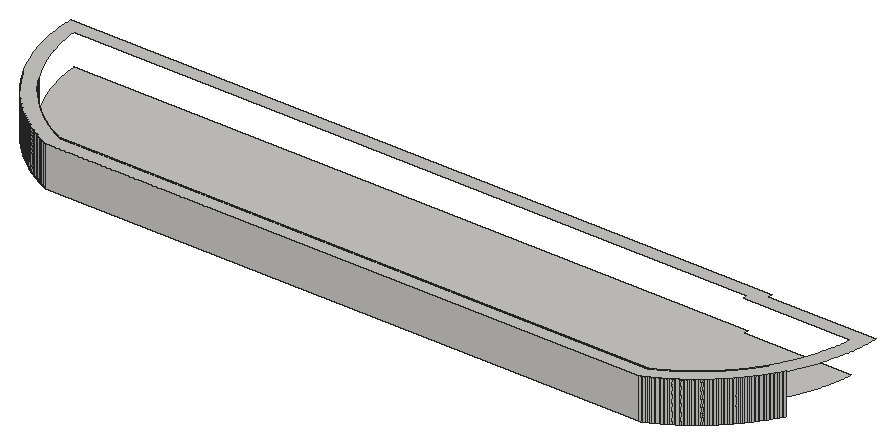
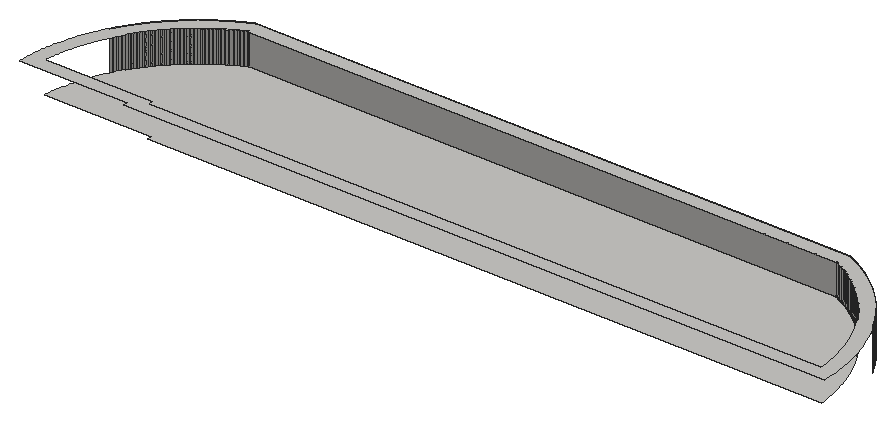
# SketchUp Ruby script. Lengths in inches.
U = 1.inch
M = Sketchup.active_model
def pt(a) = Geom::Point3d.new(a.map { |v| v * U })
def face(e, loops, mat)
  f = e.add_face(loops[0].map { |a| pt(a) })
  loops[1..].each { |l| e.add_face(l.map { |a| pt(a) }).erase! }
  f.material = f.back_material = mat if mat
  f
end
# faces: each face lists its corners as indices into pts; further lists are holes
def faces(e, pts, list, mat = nil) = list.each { |f| face(e, (f[0].is_a?(Array) ? f : [f]).map { |l| l.map { |i| pts[i] } }, mat) }
# xy, xz, yz: faces in a plane at the given z, y or x. An outline is a flat list of corners, or four numbers for a rectangle; further outlines are holes
def ring(l) = l.size == 4 ? [[l[0], l[1]], [l[2], l[1]], [l[2], l[3]], [l[0], l[3]]] : l.each_slice(2).to_a
def flat(e, list, mat, &to3) = list.each { |f| face(e, (f[0].is_a?(Array) ? f : [f]).map { |l| ring(l).map { |u, v| to3.(u, v) } }, mat) }
def xy(e, z, list, mat = nil) = flat(e, list, mat) { |x, y| [x, y, z] }
def xz(e, y, list, mat = nil) = flat(e, list, mat) { |x, z| [x, y, z] }
def yz(e, x, list, mat = nil) = flat(e, list, mat) { |y, z| [x, y, z] }
def lines(e, pts, list) = list.each { |a, b| e.add_line(pt(pts[a]), pt(pts[b])) }
# prism: a flat outline (further loops are holes) pulled along v
def prism(e, loops, v, mat = nil)
  f = face(e, loops, mat); d = Geom::Vector3d.new(v.map { |x| x * U })
  f.pushpull(f.normal.samedirection?(d) ? d.length : -d.length)
end
def box(e, o, s, mat = nil) = prism(e, [[o, [o[0] + s[0], o[1], o[2]], [o[0] + s[0], o[1] + s[1], o[2]], [o[0], o[1] + s[1], o[2]]]], [0, 0, s[2]], mat)
def at(x, y, z, deg = 0) = Geom::Transformation.translation(pt([x, y, z])) * Geom::Transformation.rotation(ORIGIN, Z_AXIS, deg.degrees)
def axes(o, x, y, z) = Geom::Transformation.new([*x, 0, *y, 0, *z, 0, *pt(o).to_a, 1])
def part(name) = M.definitions.add(name)
# library, detail: a bought-in or finely detailed component or shape, given as its bounding box
def library(name, o, s) = part(name).tap { |d| box(d.entities, o, s) }
def detail(e, o, s) = box(e.add_group.entities, o, s)
def put(e, d, t, mat = nil) = e.add_instance(d, t).tap { |i| i.material = mat if mat }
def group(e, t, mat = nil) = e.add_group.tap { |g| g.transformation = t; g.material = mat if mat }.entities
root = M.entities
M.materials.add("[Stone Sandstone Ashlar Light]").color = [201, 199, 196]
xy(root,-10,[[240.65,3,371.35,3,371.43,3.04,371.76,3.19,372.4,3.51,372.72,3.68,373.04,3.84,373.36,4.01,373.67,4.1875,373.99,4.36,374.61,4.72,375.23,5.1,375.83,5.48,376.14,5.68,376.43,5.875,376.73,6.08,377.03,6.28,377.61,6.7,377.9,6.92,378.19,7.13,378.48,7.35,378.76,7.57,379.6,8.26,380.14,8.72,380.95,9.44,381.21,9.69,381.47,9.9375,381.73,10.1875,381.98,10.44,382.24,10.7,382.74,11.22,382.98,11.48,383.23,11.74,383.71,12.28,383.94,12.55,384.17,12.83,384.4,13.1,384.86,13.66,385.08,13.94,385.52,14.52,385.73,14.8,385.94,15.1,386.36,15.68,386.96,16.58,387.15,16.88,387.34,17.1875,387.53,17.5,387.72,17.8,387.9,18.11,388.08,18.43,388.26,18.74,388.43,19.05,388.77,19.69,389.25,20.65,389.41,20.98,389.56,21.31,389.71,21.63,389.85,21.96,390,22.29,390.14,22.625,390.27,22.96,390.41,23.29,390.54,23.625,390.66,23.96,390.79,24.3,390.91,24.64,391.02,24.98,391.14,25.32,391.25,25.67,391.35,26.01,391.46,26.35,391.66,27.05,391.75,27.39,391.93,28.09,392.17,29.14,392.24,29.49,392.3125,29.85,392.38,30.2,392.44,30.56,392.5,30.91,392.56,31.27,392.61,31.62,392.66,31.98,392.71,32.33,392.75,32.69,392.79,33,369,33,369,34,219.12,34,219.14,33.77,219.17,33.41,219.29,32.33,219.34,31.98,219.39,31.62,219.44,31.27,219.5,30.91,219.56,30.56,219.62,30.2,219.6875,29.85,219.76,29.49,219.83,29.14,220.07,28.09,220.25,27.39,220.34,27.05,220.54,26.35,220.65,26.01,220.75,25.67,220.86,25.32,220.98,24.98,221.09,24.64,221.21,24.3,221.34,23.96,221.46,23.625,221.59,23.29,221.73,22.96,221.86,22.625,222,22.29,222.15,21.96,222.29,21.63,222.44,21.31,222.59,20.98,222.75,20.65,223.23,19.69,223.57,19.05,223.74,18.74,223.92,18.43,224.1,18.11,224.28,17.8,224.47,17.5,224.66,17.1875,224.85,16.88,225.04,16.58,225.64,15.68,226.06,15.1,226.27,14.8,226.48,14.52,226.92,13.94,227.14,13.66,227.6,13.1,227.83,12.83,228.06,12.55,228.29,12.28,228.77,11.74,229.02,11.48,229.26,11.22,229.76,10.7,230.02,10.44,230.27,10.1875,230.53,9.9375,230.79,9.69,231.05,9.44,231.86,8.72,232.4,8.26,233.24,7.57,233.52,7.35,233.81,7.13,234.1,6.92,234.39,6.7,234.97,6.28,235.27,6.08,235.57,5.875,235.86,5.68,236.17,5.48,236.77,5.1,237.39,4.72,238.01,4.36,238.33,4.1875,238.64,4.01,238.96,3.84,239.28,3.68,239.6,3.51,240.24,3.19,240.57,3.04]],"[Stone Sandstone Ashlar Light]")
xy(root,-3,[[[240,0,372,0,372.35,0.16,372.71,0.32,373.41,0.66,373.75,0.83,374.1,1.01,374.44,1.19,374.79,1.375,375.47,1.75,375.8,1.95,376.14,2.14,376.8,2.54,377.79,3.17,379.07,4.05,379.38,4.28,379.7,4.51,380.01,4.74,380.3125,4.98,380.62,5.22,380.92,5.46,381.82,6.21,382.11,6.46,382.41,6.72,382.69,6.98,382.98,7.24,383.27,7.51,383.55,7.77,384.1,8.32,384.375,8.59,384.65,8.87,384.92,9.15,385.18,9.4375,385.44,9.72,385.96,10.3,386.22,10.6,386.47,10.89,386.72,11.19,386.96,11.49,387.21,11.79,387.45,12.1,387.68,12.41,387.92,12.72,388.38,13.34,388.6,13.66,388.83,13.98,389.05,14.3,389.47,14.95,389.68,15.28,389.89,15.6,390.09,15.9375,390.3,16.27,390.49,16.6,390.6875,16.94,390.88,17.28,391.06,17.62,391.25,17.96,391.43,18.31,391.61,18.65,392.12,19.7,392.28,20.05,392.45,20.4,392.6,20.76,392.76,21.12,392.91,21.47,393.05,21.83,393.2,22.2,393.48,22.92,393.61,23.29,393.74,23.65,393.86,24.02,393.99,24.39,394.11,24.76,394.33,25.5,394.55,26.25,394.75,27,394.93,27.76,395.02,28.13,395.18,28.89,395.26,29.28,395.4,30.04,395.46,30.42,395.52,30.81,395.58,31.19,395.64,31.58,395.69,31.96,395.73,32.35,395.77,32.73,395.8125,33.12,395.85,33.51,395.88,33.89,395.91,34.28,395.97,35.45,395.98,35.83,395.99,36,372,36,372,37,216,37,216,36.61,216.02,35.83,216.03,35.45,216.09,34.28,216.12,33.89,216.15,33.51,216.1875,33.12,216.23,32.73,216.27,32.35,216.31,31.96,216.36,31.58,216.42,31.19,216.48,30.81,216.54,30.42,216.6,30.04,216.74,29.28,216.82,28.89,216.98,28.13,217.07,27.76,217.25,27,217.45,26.25,217.67,25.5,217.89,24.76,218.01,24.39,218.14,24.02,218.26,23.65,218.39,23.29,218.52,22.92,218.8,22.2,218.95,21.83,219.09,21.47,219.24,21.12,219.4,20.76,219.55,20.4,219.72,20.05,219.88,19.7,220.39,18.65,220.57,18.31,220.75,17.96,220.94,17.62,221.12,17.28,221.3125,16.94,221.51,16.6,221.7,16.27,221.91,15.9375,222.11,15.6,222.32,15.28,222.53,14.95,222.95,14.3,223.17,13.98,223.4,13.66,223.62,13.34,224.08,12.72,224.32,12.41,224.55,12.1,224.79,11.79,225.04,11.49,225.28,11.19,225.53,10.89,225.78,10.6,226.04,10.3,226.56,9.72,226.82,9.4375,227.08,9.15,227.35,8.87,227.625,8.59,227.9,8.32,228.45,7.77,228.73,7.51,229.02,7.24,229.31,6.98,229.59,6.72,229.89,6.46,230.18,6.21,231.08,5.46,231.38,5.22,231.6875,4.98,231.99,4.74,232.3,4.51,232.62,4.28,232.93,4.05,234.21,3.17,235.2,2.54,235.86,2.14,236.2,1.95,236.53,1.75,237.21,1.375,237.56,1.19,237.9,1.01,238.25,0.83,238.59,0.66,239.29,0.32,239.65,0.16],[240.65,3,240.57,3.04,240.24,3.19,239.6,3.51,239.28,3.68,238.96,3.84,238.64,4.01,238.33,4.1875,238.01,4.36,237.39,4.72,236.77,5.1,236.17,5.48,235.86,5.68,235.57,5.875,235.27,6.08,234.97,6.28,234.39,6.7,234.1,6.92,233.81,7.13,233.52,7.35,233.24,7.57,232.4,8.26,231.86,8.72,231.05,9.44,230.79,9.69,230.53,9.9375,230.27,10.1875,230.02,10.44,229.76,10.7,229.26,11.22,229.02,11.48,228.77,11.74,228.29,12.28,228.06,12.55,227.83,12.83,227.6,13.1,227.14,13.66,226.92,13.94,226.48,14.52,226.27,14.8,226.06,15.1,225.64,15.68,225.04,16.58,224.85,16.88,224.66,17.1875,224.47,17.5,224.28,17.8,224.1,18.11,223.92,18.43,223.74,18.74,223.57,19.05,223.23,19.69,222.75,20.65,222.59,20.98,222.44,21.31,222.29,21.63,222.15,21.96,222,22.29,221.86,22.625,221.73,22.96,221.59,23.29,221.46,23.625,221.34,23.96,221.21,24.3,221.09,24.64,220.98,24.98,220.86,25.32,220.75,25.67,220.65,26.01,220.54,26.35,220.34,27.05,220.25,27.39,220.07,28.09,219.83,29.14,219.76,29.49,219.6875,29.85,219.62,30.2,219.56,30.56,219.5,30.91,219.44,31.27,219.39,31.62,219.34,31.98,219.29,32.33,219.17,33.41,219.14,33.77,219.12,34,369,34,369,33,392.79,33,392.75,32.69,392.71,32.33,392.66,31.98,392.61,31.62,392.56,31.27,392.5,30.91,392.44,30.56,392.38,30.2,392.3125,29.85,392.24,29.49,392.17,29.14,391.93,28.09,391.75,27.39,391.66,27.05,391.46,26.35,391.35,26.01,391.25,25.67,391.14,25.32,391.02,24.98,390.91,24.64,390.79,24.3,390.66,23.96,390.54,23.625,390.41,23.29,390.27,22.96,390.14,22.625,390,22.29,389.85,21.96,389.71,21.63,389.56,21.31,389.41,20.98,389.25,20.65,388.77,19.69,388.43,19.05,388.26,18.74,388.08,18.43,387.9,18.11,387.72,17.8,387.53,17.5,387.34,17.1875,387.15,16.88,386.96,16.58,386.36,15.68,385.94,15.1,385.73,14.8,385.52,14.52,385.08,13.94,384.86,13.66,384.4,13.1,384.17,12.83,383.94,12.55,383.71,12.28,383.23,11.74,382.98,11.48,382.74,11.22,382.24,10.7,381.98,10.44,381.73,10.1875,381.47,9.9375,381.21,9.69,380.95,9.44,380.14,8.72,379.6,8.26,378.76,7.57,378.48,7.35,378.19,7.13,377.9,6.92,377.61,6.7,377.03,6.28,376.73,6.08,376.43,5.875,376.14,5.68,375.83,5.48,375.23,5.1,374.61,4.72,373.99,4.36,373.67,4.1875,373.36,4.01,373.04,3.84,372.72,3.68,372.4,3.51,371.76,3.19,371.43,3.04,371.35,3]]],"[Stone Sandstone Ashlar Light]")
xz(root,0,[[240,-12,372,-3]],"[Stone Sandstone Ashlar Light]")
xz(root,3,[[240.65,-10,371.35,-3]],"[Stone Sandstone Ashlar Light]")
p = [[240,0,-3],[239.65,0.16,-3],[239.65,0.16,-12],[240,0,-12],[372.35,0.16,-3],[372,0,-3],
  [372,0,-12],[372.35,0.16,-12],[239.29,0.32,-3],[239.29,0.32,-12],[372.71,0.32,-3],[372.71,0.32,-12],
  [238.94,0.49,-3],[238.94,0.49,-12],[373.06,0.49,-3],[373.06,0.49,-12],[238.59,0.66,-3],[238.59,0.66,-12],
  [373.41,0.66,-3],[373.41,0.66,-12],[238.25,0.83,-3],[238.25,0.83,-12],[373.75,0.83,-3],[373.75,0.83,-12],
  [237.9,1.01,-3],[237.9,1.01,-12],[374.1,1.01,-3],[374.1,1.01,-12],[237.56,1.19,-3],[237.56,1.19,-12],
  [374.44,1.19,-3],[374.44,1.19,-12],[237.21,1.375,-3],[237.21,1.375,-12],[374.79,1.375,-3],[374.79,1.375,-12],
  [236.87,1.5625,-3],[236.87,1.5625,-12],[375.13,1.5625,-3],[375.13,1.5625,-12],[236.53,1.75,-3],[236.53,1.75,-12],
  [375.47,1.75,-3],[375.47,1.75,-12],[236.2,1.95,-3],[236.2,1.95,-12],[375.8,1.95,-3],[375.8,1.95,-12],
  [235.86,2.14,-3],[235.86,2.14,-12],[376.14,2.14,-3],[376.14,2.14,-12],[235.53,2.34,-3],[235.53,2.34,-12],
  [376.47,2.34,-3],[376.47,2.34,-12],[235.2,2.54,-3],[235.2,2.54,-12],[376.8,2.54,-3],[376.8,2.54,-12],
  [234.87,2.75,-3],[234.87,2.75,-12],[377.13,2.75,-3],[377.13,2.75,-12],[234.54,2.96,-3],[234.54,2.96,-12],
  [377.46,2.96,-3],[377.46,2.96,-12],[234.21,3.17,-3],[234.21,3.17,-12],[377.79,3.17,-3],[377.79,3.17,-12],
  [233.89,3.39,-3],[233.89,3.39,-12],[378.11,3.39,-3],[378.11,3.39,-12],[233.57,3.61,-3],[233.57,3.61,-12],
  [378.43,3.61,-3],[378.43,3.61,-12],[233.25,3.83,-3],[233.25,3.83,-12],[378.75,3.83,-3],[378.75,3.83,-12],
  [232.93,4.05,-3],[232.93,4.05,-12],[379.07,4.05,-3],[379.07,4.05,-12],[232.62,4.28,-3],[232.62,4.28,-12],
  [379.38,4.28,-3],[379.38,4.28,-12],[232.3,4.51,-3],[232.3,4.51,-12],[379.7,4.51,-3],[379.7,4.51,-12],
  [231.99,4.74,-3],[231.99,4.74,-12],[380.01,4.74,-3],[380.01,4.74,-12],[231.6875,4.98,-3],[231.6875,4.98,-12],
  [380.3125,4.98,-3],[380.3125,4.98,-12],[231.38,5.22,-3],[231.38,5.22,-12],[380.62,5.22,-3],[380.62,5.22,-12],
  [231.08,5.46,-3],[231.08,5.46,-12],[380.92,5.46,-3],[380.92,5.46,-12],[230.78,5.71,-3],[230.78,5.71,-12],
  [381.22,5.71,-3],[381.22,5.71,-12],[230.48,5.96,-3],[230.48,5.96,-12],[381.52,5.96,-3],[381.52,5.96,-12],
  [230.18,6.21,-3],[230.18,6.21,-12],[381.82,6.21,-3],[381.82,6.21,-12],[229.89,6.46,-3],[229.89,6.46,-12],
  [382.11,6.46,-3],[382.11,6.46,-12],[229.59,6.72,-3],[229.59,6.72,-12],[382.41,6.72,-3],[382.41,6.72,-12],
  [229.31,6.98,-3],[229.31,6.98,-12],[382.69,6.98,-3],[382.69,6.98,-12],[229.02,7.24,-3],[229.02,7.24,-12],
  [382.98,7.24,-3],[382.98,7.24,-12],[228.73,7.51,-3],[228.73,7.51,-12],[383.27,7.51,-3],[383.27,7.51,-12],
  [228.45,7.77,-3],[228.45,7.77,-12],[383.55,7.77,-3],[383.55,7.77,-12],[228.17,8.05,-3],[228.17,8.05,-12],
  [383.83,8.05,-3],[383.83,8.05,-12],[227.9,8.32,-3],[227.9,8.32,-12],[384.1,8.32,-3],[384.1,8.32,-12],
  [227.625,8.59,-3],[227.625,8.59,-12],[384.375,8.59,-3],[384.375,8.59,-12],[227.35,8.87,-3],[227.35,8.87,-12],
  [384.65,8.87,-3],[384.65,8.87,-12],[227.08,9.15,-3],[227.08,9.15,-12],[384.92,9.15,-3],[384.92,9.15,-12],
  [226.82,9.4375,-3],[226.82,9.4375,-12],[385.18,9.4375,-3],[385.18,9.4375,-12],[226.56,9.72,-3],[226.56,9.72,-12],
  [385.44,9.72,-3],[385.44,9.72,-12],[226.3,10.01,-3],[226.3,10.01,-12],[385.7,10.01,-3],[385.7,10.01,-12],
  [226.04,10.3,-3],[226.04,10.3,-12],[385.96,10.3,-3],[385.96,10.3,-12],[225.78,10.6,-3],[225.78,10.6,-12],
  [386.22,10.6,-3],[386.22,10.6,-12],[225.53,10.89,-3],[225.53,10.89,-12],[386.47,10.89,-3],[386.47,10.89,-12],
  [225.28,11.19,-3],[225.28,11.19,-12],[386.72,11.19,-3],[386.72,11.19,-12],[225.04,11.49,-3],[225.04,11.49,-12],
  [386.96,11.49,-3],[386.96,11.49,-12],[224.79,11.79,-3],[224.79,11.79,-12],[387.21,11.79,-3],[387.21,11.79,-12],
  [224.55,12.1,-3],[224.55,12.1,-12],[387.45,12.1,-3],[387.45,12.1,-12],[224.32,12.41,-3],[224.32,12.41,-12],
  [387.68,12.41,-3],[387.68,12.41,-12],[224.08,12.72,-3],[224.08,12.72,-12],[387.92,12.72,-3],[387.92,12.72,-12],
  [223.85,13.03,-3],[223.85,13.03,-12],[388.15,13.03,-3],[388.15,13.03,-12],[223.62,13.34,-3],[223.62,13.34,-12],
  [388.38,13.34,-3],[388.38,13.34,-12],[223.4,13.66,-3],[223.4,13.66,-12],[388.6,13.66,-3],[388.6,13.66,-12],
  [223.17,13.98,-3],[223.17,13.98,-12],[388.83,13.98,-3],[388.83,13.98,-12],[222.95,14.3,-3],[222.95,14.3,-12],
  [389.05,14.3,-3],[389.05,14.3,-12],[222.74,14.625,-3],[222.74,14.625,-12],[389.26,14.625,-3],[389.26,14.625,-12],
  [222.53,14.95,-3],[222.53,14.95,-12],[389.47,14.95,-3],[389.47,14.95,-12],[222.32,15.28,-3],[222.32,15.28,-12],
  [389.68,15.28,-3],[389.68,15.28,-12],[222.11,15.6,-3],[222.11,15.6,-12],[389.89,15.6,-3],[389.89,15.6,-12],
  [221.91,15.9375,-3],[221.91,15.9375,-12],[390.09,15.9375,-3],[390.09,15.9375,-12],[221.7,16.27,-3],[221.7,16.27,-12],
  [390.3,16.27,-3],[390.3,16.27,-12],[221.51,16.6,-3],[221.51,16.6,-12],[390.49,16.6,-3],[390.49,16.6,-12],
  [221.3125,16.94,-3],[221.3125,16.94,-12],[390.6875,16.94,-3],[390.6875,16.94,-12],[221.12,17.28,-3],[221.12,17.28,-12],
  [390.88,17.28,-3],[390.88,17.28,-12],[240.24,3.19,-3],[240.57,3.04,-3],[240.57,3.04,-10],[240.24,3.19,-10],
  [240.65,3,-3],[240.65,3,-10],[371.35,3,-3],[371.43,3.04,-3],[371.43,3.04,-10],[371.35,3,-10],
  [371.76,3.19,-3],[371.76,3.19,-10],[239.92,3.35,-3],[239.92,3.35,-10],[372.08,3.35,-3],[372.08,3.35,-10],
  [239.6,3.51,-3],[239.6,3.51,-10],[372.4,3.51,-3],[372.4,3.51,-10],[239.28,3.68,-3],[239.28,3.68,-10],
  [372.72,3.68,-3],[372.72,3.68,-10],[238.96,3.84,-3],[238.96,3.84,-10],[373.04,3.84,-3],[373.04,3.84,-10],
  [238.64,4.01,-3],[238.64,4.01,-10],[373.36,4.01,-3],[373.36,4.01,-10],[238.33,4.1875,-3],[238.33,4.1875,-10],
  [373.67,4.1875,-3],[373.67,4.1875,-10],[238.01,4.36,-3],[238.01,4.36,-10],[373.99,4.36,-3],[373.99,4.36,-10],
  [237.7,4.54,-3],[237.7,4.54,-10],[374.3,4.54,-3],[374.3,4.54,-10],[237.39,4.72,-3],[237.39,4.72,-10],
  [374.61,4.72,-3],[374.61,4.72,-10],[237.08,4.91,-3],[237.08,4.91,-10],[374.92,4.91,-3],[374.92,4.91,-10],
  [236.77,5.1,-3],[236.77,5.1,-10],[375.23,5.1,-3],[375.23,5.1,-10],[236.47,5.29,-3],[236.47,5.29,-10],
  [375.53,5.29,-3],[375.53,5.29,-10],[236.17,5.48,-3],[236.17,5.48,-10],[375.83,5.48,-3],[375.83,5.48,-10],
  [235.86,5.68,-3],[235.86,5.68,-10],[376.14,5.68,-3],[376.14,5.68,-10],[235.57,5.875,-3],[235.57,5.875,-10],
  [376.43,5.875,-3],[376.43,5.875,-10],[235.27,6.08,-3],[235.27,6.08,-10],[376.73,6.08,-3],[376.73,6.08,-10],
  [234.97,6.28,-3],[234.97,6.28,-10],[377.03,6.28,-3],[377.03,6.28,-10],[234.68,6.49,-3],[234.68,6.49,-10],
  [377.32,6.49,-3],[377.32,6.49,-10],[234.39,6.7,-3],[234.39,6.7,-10],[377.61,6.7,-3],[377.61,6.7,-10],
  [234.1,6.92,-3],[234.1,6.92,-10],[377.9,6.92,-3],[377.9,6.92,-10],[233.81,7.13,-3],[233.81,7.13,-10],
  [378.19,7.13,-3],[378.19,7.13,-10],[233.52,7.35,-3],[233.52,7.35,-10],[378.48,7.35,-3],[378.48,7.35,-10],
  [233.24,7.57,-3],[233.24,7.57,-10],[378.76,7.57,-3],[378.76,7.57,-10],[232.96,7.8,-3],[232.96,7.8,-10],
  [379.04,7.8,-3],[379.04,7.8,-10],[232.68,8.03,-3],[232.68,8.03,-10],[379.32,8.03,-3],[379.32,8.03,-10],
  [232.4,8.26,-3],[232.4,8.26,-10],[379.6,8.26,-3],[379.6,8.26,-10],[232.13,8.49,-3],[232.13,8.49,-10],
  [379.87,8.49,-3],[379.87,8.49,-10],[231.86,8.72,-3],[231.86,8.72,-10],[380.14,8.72,-3],[380.14,8.72,-10],
  [231.59,8.96,-3],[231.59,8.96,-10],[380.41,8.96,-3],[380.41,8.96,-10],[231.32,9.2,-3],[231.32,9.2,-10],
  [380.68,9.2,-3],[380.68,9.2,-10],[231.05,9.44,-3],[231.05,9.44,-10],[380.95,9.44,-3],[380.95,9.44,-10],
  [230.79,9.69,-3],[230.79,9.69,-10],[381.21,9.69,-3],[381.21,9.69,-10],[230.53,9.9375,-3],[230.53,9.9375,-10],
  [381.47,9.9375,-3],[381.47,9.9375,-10],[230.27,10.1875,-3],[230.27,10.1875,-10],[381.73,10.1875,-3],[381.73,10.1875,-10],
  [230.02,10.44,-3],[230.02,10.44,-10],[381.98,10.44,-3],[381.98,10.44,-10],[229.76,10.7,-3],[229.76,10.7,-10],
  [382.24,10.7,-3],[382.24,10.7,-10],[229.51,10.96,-3],[229.51,10.96,-10],[382.49,10.96,-3],[382.49,10.96,-10],
  [229.26,11.22,-3],[229.26,11.22,-10],[382.74,11.22,-3],[382.74,11.22,-10],[229.02,11.48,-3],[229.02,11.48,-10],
  [382.98,11.48,-3],[382.98,11.48,-10],[228.77,11.74,-3],[228.77,11.74,-10],[383.23,11.74,-3],[383.23,11.74,-10],
  [228.53,12.01,-3],[228.53,12.01,-10],[383.47,12.01,-3],[383.47,12.01,-10],[228.29,12.28,-3],[228.29,12.28,-10],
  [383.71,12.28,-3],[383.71,12.28,-10],[228.06,12.55,-3],[228.06,12.55,-10],[383.94,12.55,-3],[383.94,12.55,-10],
  [227.83,12.83,-3],[227.83,12.83,-10],[384.17,12.83,-3],[384.17,12.83,-10],[227.6,13.1,-3],[227.6,13.1,-10],
  [384.4,13.1,-3],[384.4,13.1,-10],[227.37,13.38,-3],[227.37,13.38,-10],[384.63,13.38,-3],[384.63,13.38,-10],
  [227.14,13.66,-3],[227.14,13.66,-10],[384.86,13.66,-3],[384.86,13.66,-10],[226.92,13.94,-3],[226.92,13.94,-10],
  [385.08,13.94,-3],[385.08,13.94,-10],[226.7,14.23,-3],[226.7,14.23,-10],[385.3,14.23,-3],[385.3,14.23,-10],
  [226.48,14.52,-3],[226.48,14.52,-10],[385.52,14.52,-3],[385.52,14.52,-10],[226.27,14.8,-3],[226.27,14.8,-10],
  [385.73,14.8,-3],[385.73,14.8,-10],[226.06,15.1,-3],[226.06,15.1,-10],[385.94,15.1,-3],[385.94,15.1,-10],
  [225.85,15.39,-3],[225.85,15.39,-10],[386.15,15.39,-3],[386.15,15.39,-10],[225.64,15.68,-3],[225.64,15.68,-10],
  [386.36,15.68,-3],[386.36,15.68,-10],[225.44,15.98,-3],[225.44,15.98,-10],[386.56,15.98,-3],[386.56,15.98,-10],
  [225.24,16.28,-3],[225.24,16.28,-10],[386.76,16.28,-3],[386.76,16.28,-10],[225.04,16.58,-3],[225.04,16.58,-10],
  [386.96,16.58,-3],[386.96,16.58,-10],[224.85,16.88,-3],[224.85,16.88,-10],[387.15,16.88,-3],[387.15,16.88,-10],
  [224.66,17.1875,-3],[224.66,17.1875,-10],[387.34,17.1875,-3],[387.34,17.1875,-10]]
faces(root,p,[[0,1,2,3],[4,5,6,7],[1,8,9,2],[10,4,7,11],[8,12,13,9],[14,10,11,15],[12,16,17,13],[18,14,15,19],
  [16,20,21,17],[22,18,19,23],[20,24,25,21],[26,22,23,27],[24,28,29,25],[30,26,27,31],[28,32,33,29],[34,30,31,35],
  [32,36,37,33],[38,34,35,39],[36,40,41,37],[42,38,39,43],[40,44,45,41],[46,42,43,47],[44,48,49,45],[50,46,47,51],
  [48,52,53,49],[54,50,51,55],[52,56,57,53],[58,54,55,59],[56,60,61,57],[62,58,59,63],[60,64,65,61],[66,62,63,67],
  [64,68,69,65],[70,66,67,71],[68,72,73,69],[74,70,71,75],[72,76,77,73],[78,74,75,79],[76,80,81,77],[82,78,79,83],
  [80,84,85,81],[86,82,83,87],[84,88,89,85],[90,86,87,91],[88,92,93,89],[94,90,91,95],[92,96,97,93],[98,94,95,99],
  [96,100,101,97],[102,98,99,103],[100,104,105,101],[106,102,103,107],[104,108,109,105],[110,106,107,111],[108,112,113,109],[114,110,111,115],
  [112,116,117,113],[118,114,115,119],[116,120,121,117],[122,118,119,123],[120,124,125,121],[126,122,123,127],[124,128,129,125],[130,126,127,131],
  [128,132,133,129],[134,130,131,135],[132,136,137,133],[138,134,135,139],[136,140,141,137],[142,138,139,143],[140,144,145,141],[146,142,143,147],
  [144,148,149,145],[150,146,147,151],[148,152,153,149],[154,150,151,155],[152,156,157,153],[158,154,155,159],[156,160,161,157],[162,158,159,163],
  [160,164,165,161],[166,162,163,167],[164,168,169,165],[170,166,167,171],[168,172,173,169],[174,170,171,175],[172,176,177,173],[178,174,175,179],
  [176,180,181,177],[182,178,179,183],[180,184,185,181],[186,182,183,187],[184,188,189,185],[190,186,187,191],[188,192,193,189],[194,190,191,195],
  [192,196,197,193],[198,194,195,199],[196,200,201,197],[202,198,199,203],[200,204,205,201],[206,202,203,207],[204,208,209,205],[210,206,207,211],
  [208,212,213,209],[214,210,211,215],[212,216,217,213],[218,214,215,219],[216,220,221,217],[222,218,219,223],[220,224,225,221],[226,222,223,227],
  [224,228,229,225],[230,226,227,231],[228,232,233,229],[234,230,231,235],[232,236,237,233],[238,234,235,239],[236,240,241,237],[242,238,239,243],
  [240,244,245,241],[246,242,243,247],[244,248,249,245],[250,246,247,251],[248,252,253,249],[254,250,251,255],[252,256,257,253],[258,254,255,259],
  [256,260,261,257],[262,258,259,263],[260,264,265,261],[266,262,263,267],[264,268,269,265],[270,266,267,271],[272,273,274,275],[273,276,277,274],
  [278,279,280,281],[279,282,283,280],[284,272,275,285],[282,286,287,283],[288,284,285,289],[286,290,291,287],[292,288,289,293],[290,294,295,291],
  [296,292,293,297],[294,298,299,295],[300,296,297,301],[298,302,303,299],[304,300,301,305],[302,306,307,303],[308,304,305,309],[306,310,311,307],
  [312,308,309,313],[310,314,315,311],[316,312,313,317],[314,318,319,315],[320,316,317,321],[318,322,323,319],[324,320,321,325],[322,326,327,323],
  [328,324,325,329],[326,330,331,327],[332,328,329,333],[330,334,335,331],[336,332,333,337],[334,338,339,335],[340,336,337,341],[338,342,343,339],
  [344,340,341,345],[342,346,347,343],[348,344,345,349],[346,350,351,347],[352,348,349,353],[350,354,355,351],[356,352,353,357],[354,358,359,355],
  [360,356,357,361],[358,362,363,359],[364,360,361,365],[362,366,367,363],[368,364,365,369],[366,370,371,367],[372,368,369,373],[370,374,375,371],
  [376,372,373,377],[374,378,379,375],[380,376,377,381],[378,382,383,379],[384,380,381,385],[382,386,387,383],[388,384,385,389],[386,390,391,387],
  [392,388,389,393],[390,394,395,391],[396,392,393,397],[394,398,399,395],[400,396,397,401],[398,402,403,399],[404,400,401,405],[402,406,407,403],
  [408,404,405,409],[406,410,411,407],[412,408,409,413],[410,414,415,411],[416,412,413,417],[414,418,419,415],[420,416,417,421],[418,422,423,419],
  [424,420,421,425],[422,426,427,423],[428,424,425,429],[426,430,431,427],[432,428,429,433],[430,434,435,431],[436,432,433,437],[434,438,439,435],
  [440,436,437,441],[438,442,443,439],[444,440,441,445],[442,446,447,443],[448,444,445,449],[446,450,451,447],[452,448,449,453],[450,454,455,451],
  [456,452,453,457],[454,458,459,455],[460,456,457,461],[458,462,463,459],[464,460,461,465],[462,466,467,463],[468,464,465,469],[466,470,471,467],
  [472,468,469,473],[470,474,475,471],[476,472,473,477],[474,478,479,475],[480,476,477,481],[478,482,483,479],[484,480,481,485],[482,486,487,483],
  [488,484,485,489],[486,490,491,487],[492,488,489,493],[490,494,495,491],[496,492,493,497],[494,498,499,495],[500,496,497,501],[498,502,503,499],
  [504,500,501,505],[502,506,507,503],[508,504,505,509],[506,510,511,507],[512,508,509,513],[510,514,515,511],[516,512,513,517],[514,518,519,515]],"[Stone Sandstone Ashlar Light]")
